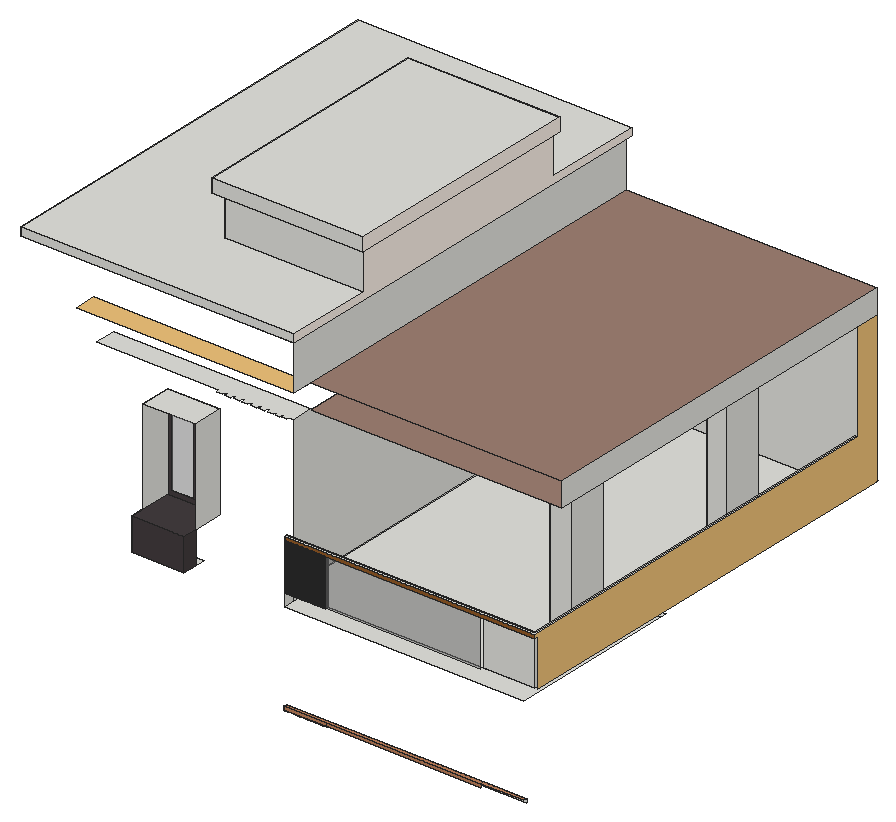
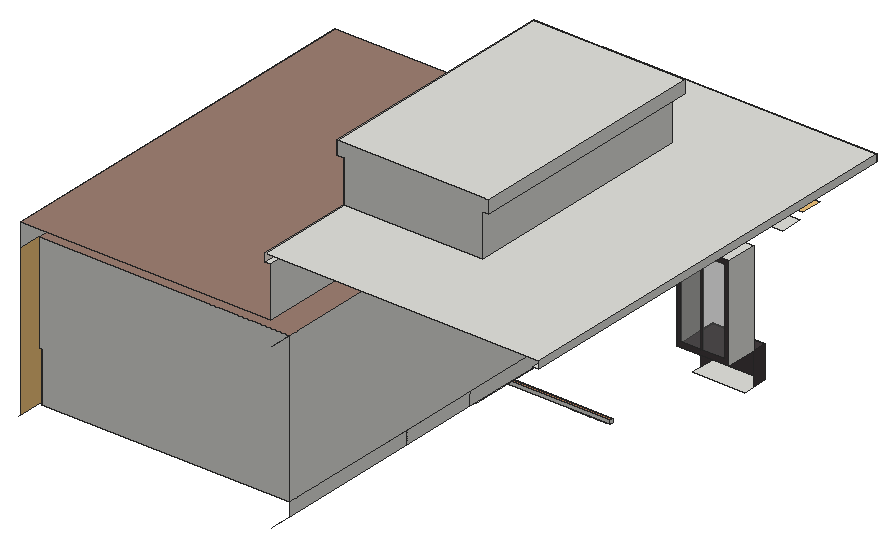
# SketchUp Ruby script. Lengths in inches.
U = 1.inch
M = Sketchup.active_model
def pt(a) = Geom::Point3d.new(a.map { |v| v * U })
def face(e, loops, mat)
  f = e.add_face(loops[0].map { |a| pt(a) })
  loops[1..].each { |l| e.add_face(l.map { |a| pt(a) }).erase! }
  f.material = f.back_material = mat if mat
  f
end
# faces: each face lists its corners as indices into pts; further lists are holes
def faces(e, pts, list, mat = nil) = list.each { |f| face(e, (f[0].is_a?(Array) ? f : [f]).map { |l| l.map { |i| pts[i] } }, mat) }
# xy, xz, yz: faces in a plane at the given z, y or x. An outline is a flat list of corners, or four numbers for a rectangle; further outlines are holes
def ring(l) = l.size == 4 ? [[l[0], l[1]], [l[2], l[1]], [l[2], l[3]], [l[0], l[3]]] : l.each_slice(2).to_a
def flat(e, list, mat, &to3) = list.each { |f| face(e, (f[0].is_a?(Array) ? f : [f]).map { |l| ring(l).map { |u, v| to3.(u, v) } }, mat) }
def xy(e, z, list, mat = nil) = flat(e, list, mat) { |x, y| [x, y, z] }
def xz(e, y, list, mat = nil) = flat(e, list, mat) { |x, z| [x, y, z] }
def yz(e, x, list, mat = nil) = flat(e, list, mat) { |y, z| [x, y, z] }
def lines(e, pts, list) = list.each { |a, b| e.add_line(pt(pts[a]), pt(pts[b])) }
# prism: a flat outline (further loops are holes) pulled along v
def prism(e, loops, v, mat = nil)
  f = face(e, loops, mat); d = Geom::Vector3d.new(v.map { |x| x * U })
  f.pushpull(f.normal.samedirection?(d) ? d.length : -d.length)
end
def box(e, o, s, mat = nil) = prism(e, [[o, [o[0] + s[0], o[1], o[2]], [o[0] + s[0], o[1] + s[1], o[2]], [o[0], o[1] + s[1], o[2]]]], [0, 0, s[2]], mat)
def at(x, y, z, deg = 0) = Geom::Transformation.translation(pt([x, y, z])) * Geom::Transformation.rotation(ORIGIN, Z_AXIS, deg.degrees)
def axes(o, x, y, z) = Geom::Transformation.new([*x, 0, *y, 0, *z, 0, *pt(o).to_a, 1])
def part(name) = M.definitions.add(name)
# library, detail: a bought-in or finely detailed component or shape, given as its bounding box
def library(name, o, s) = part(name).tap { |d| box(d.entities, o, s) }
def detail(e, o, s) = box(e.add_group.entities, o, s)
def put(e, d, t, mat = nil) = e.add_instance(d, t).tap { |i| i.material = mat if mat }
def group(e, t, mat = nil) = e.add_group.tap { |g| g.transformation = t; g.material = mat if mat }.entities
root = M.entities
M.materials.add("Niraj_Skin").color = [158, 128, 115]
M.materials.add("[0009_Linen]").color = [250, 240, 230]
M.materials.add("[Asphalt New]").color = [67, 60, 62]
M.materials.add("[Translucent Glass Gray]").color = [128, 128, 128]
M.materials["[Translucent Glass Gray]"].alpha = 0.5
M.materials.add("[Wood Floor Parquet]").color = [145, 89, 39]
M.materials.add("[Wood OSB]").color = [240, 195, 122]
M.materials.add("[Wood Veneer 02]").color = [190, 128, 91]
xy(root,232.0625,[[228.72,126.77,231.29,127.27],[231.29,126.77,231.72,129.76],[231.72,126.77,233.04,127.39],[233.04,126.77,233.47,129.76],[233.47,126.77,234.79,127.46],
  [234.79,126.77,235.22,129.76],[235.22,126.77,236.54,127.64],[236.54,126.77,236.97,129.76],[236.97,126.77,238.29,127.46],[238.29,126.77,238.72,129.76],
  [238.72,126.77,240.04,127.64],[240.04,126.77,240.47,129.76],[240.47,126.77,241.79,127.33],[241.79,126.77,242.22,129.76],[242.22,126.77,243.54,127.27],
  [243.54,126.77,243.97,129.76],[243.97,126.77,245.29,127.27],[245.29,126.77,245.72,129.76],[245.72,126.77,247.04,127.27],[247.04,126.77,247.54,129.76],
  [247.54,126.77,248.85,127.27],[248.85,126.77,249.35,129.76],[249.35,126.77,250.67,127.27],[250.67,126.77,251.16,129.76],[251.16,126.77,252.48,127.27],
  [252.48,126.77,252.97,129.76],[252.97,126.77,254.29,127.27],[254.29,126.77,254.79,129.76],[254.79,126.77,256.1,127.27],[256.1,126.77,256.6,129.76],
  [256.6,126.77,257.92,127.27],[257.92,126.77,258.41,129.76],[258.41,126.77,259.73,127.27],[259.73,126.77,260.22,129.76],[260.22,126.77,261.54,127.27],
  [261.54,126.77,262.04,129.76],[262.04,126.77,263.35,127.27],[263.35,126.77,263.85,129.76],[263.85,126.77,265.17,127.27],[228.72,127.27,228.75,129.76],
  [228.75,127.27,231.29,129.76],[242.22,127.27,243.54,129.76],[243.97,127.27,245.29,129.76],[245.72,127.27,247.04,129.76],[247.54,127.27,248.85,129.76],
  [249.35,127.27,250.67,129.76],[251.16,127.27,252.48,129.76],[252.97,127.27,254.29,129.76],[254.79,127.27,256.1,129.76],[256.6,127.27,257.92,129.76],
  [258.41,127.27,259.73,129.76],[260.22,127.27,261.54,129.76],[262.04,127.27,263.35,129.76],[240.47,127.33,241.79,129.76],[231.72,127.39,233.04,129.76],
  [233.47,127.46,234.79,129.76],[236.97,127.46,238.29,129.76],[235.22,127.64,236.54,129.76],[238.72,127.64,240.04,129.76]])
xy(root,235.06,[[228.72,126.77,396.96,129.76],[396.96,126.77,433.38,129.76]],"[Wood Veneer 02]")
xy(root,308.65,[[99.93,124.58,144.79,146.21]])
xy(root,311.125,[[228.75,126.77,433.38,272.95],[227.87,136.77,228.75,176.35],[227.87,176.35,228.75,272.95],[228.75,272.95,433.38,278.53]])
xy(root,322.1875,[[228.75,126.77,229.82,127.39],[229.82,126.77,230.22,129.24],[230.22,126.77,230.99,127.39],[230.99,126.77,231.28,129.24],[231.28,126.77,232.05,127.39],
  [232.05,126.77,232.34,129.24],[232.34,126.77,233.11,127.39],[233.11,126.77,233.4,129.24],[233.4,126.77,234.17,127.39],[234.17,126.77,234.47,129.24],
  [234.47,126.77,235.24,127.39],[235.24,126.77,235.53,129.24],[235.53,126.77,236.3,127.39],[236.3,126.77,236.59,129.24],[236.59,126.77,237.36,127.39],
  [237.36,126.77,237.65,129.24],[237.65,126.77,238.42,127.39],[238.42,126.77,238.72,129.24],[238.72,126.77,239.49,127.39],[239.49,126.77,239.78,129.24],
  [239.78,126.77,240.55,127.39],[240.55,126.77,240.84,129.24],[240.84,126.77,241.61,127.39],[241.61,126.77,241.9,129.24],[241.9,126.77,242.67,127.39],
  [242.67,126.77,242.97,129.24],[242.97,126.77,243.74,127.39],[243.74,126.77,244.03,129.24],[244.03,126.77,244.8,127.39],[244.8,126.77,245.09,129.24],
  [245.09,126.77,245.86,127.39],[245.86,126.77,246.15,129.24],[246.15,126.77,246.92,127.39],[246.92,126.77,247.22,129.24],[247.22,126.77,247.99,127.39],
  [247.99,126.77,248.28,129.24],[248.28,126.77,249.05,127.39],[249.05,126.77,249.34,129.24],[249.34,126.77,250.11,127.39],[250.11,126.77,250.4,129.24],
  [250.4,126.77,251.17,127.39],[251.17,126.77,251.47,129.24],[251.47,126.77,252.24,127.39],[252.24,126.77,252.72,129.24],[252.72,126.77,253.49,127.39],
  [253.49,126.77,253.84,129.24],[253.84,126.77,254.61,127.39],[254.61,126.77,255.15,129.24],[255.15,126.77,255.92,127.14],[255.92,126.77,256.4,129.24],
  [256.4,126.77,257.17,127.14],[257.17,126.77,257.78,129.24],[257.78,126.77,258.55,127.14],[258.55,126.77,259.15,129.24],[259.15,126.77,259.92,127.14],
  [259.92,126.77,260.53,129.24],[260.53,126.77,261.3,127.14],[261.3,126.77,261.9,129.24],[261.9,126.77,262.67,127.14],[262.67,126.77,263.28,129.24],
  [255.15,127.14,255.92,129.24],[256.4,127.14,257.17,129.24],[257.78,127.14,258.55,129.24],[259.15,127.14,259.92,129.24],[260.53,127.14,261.3,129.24],
  [261.9,127.14,262.67,129.24],[230.22,127.39,230.99,129.24],[231.28,127.39,232.05,129.24],[232.34,127.39,233.11,129.24],[233.4,127.39,234.17,129.24],
  [234.47,127.39,235.24,129.24],[235.53,127.39,236.3,129.24],[236.59,127.39,237.36,129.24],[237.65,127.39,238.42,129.24],[238.72,127.39,239.49,129.24],
  [239.78,127.39,240.55,129.24],[240.84,127.39,241.61,129.24],[241.9,127.39,242.67,129.24],[242.97,127.39,243.74,129.24],[244.03,127.39,244.8,129.24],
  [245.09,127.39,245.86,129.24],[246.15,127.39,246.92,129.24],[247.22,127.39,247.99,129.24],[248.28,127.39,249.05,129.24],[249.34,127.39,250.11,129.24],
  [250.4,127.39,251.17,129.24],[251.47,127.39,252.24,129.24],[252.72,127.39,253.49,129.24],[253.84,127.39,254.61,129.24],[[228.75,129.24,440.6,471.23],[402.85,193.05,421.1,226.3],[404.6,358.3,421.1,391.55]]])
xy(root,336.38,[[99.93,124.58,144.79,163.21]],"[Asphalt New]")
xy(root,361.9375,[[228.75,126.77,229.82,127.39],[229.82,126.77,230.22,129.24],[230.22,126.77,230.99,127.39],[230.99,126.77,231.28,129.24],[231.28,126.77,232.05,127.39],
  [232.05,126.77,232.34,129.24],[232.34,126.77,233.11,127.39],[233.11,126.77,233.4,129.24],[233.4,126.77,234.17,127.39],[234.17,126.77,234.47,129.24],
  [234.47,126.77,235.24,127.39],[235.24,126.77,235.53,129.24],[235.53,126.77,236.3,127.39],[236.3,126.77,236.59,129.24],[236.59,126.77,237.36,127.39],
  [237.36,126.77,237.65,129.24],[237.65,126.77,238.42,127.39],[238.42,126.77,238.72,129.24],[238.72,126.77,239.49,127.39],[239.49,126.77,239.78,129.24],
  [239.78,126.77,240.55,127.39],[240.55,126.77,240.84,129.24],[240.84,126.77,241.61,127.39],[241.61,126.77,241.9,129.24],[241.9,126.77,242.67,127.39],
  [242.67,126.77,242.97,129.24],[242.97,126.77,243.74,127.39],[243.74,126.77,244.03,129.24],[244.03,126.77,244.8,127.39],[244.8,126.77,245.09,129.24],
  [245.09,126.77,245.86,127.39],[245.86,126.77,246.15,129.24],[246.15,126.77,246.92,127.39],[246.92,126.77,247.22,129.24],[247.22,126.77,247.99,127.39],
  [247.99,126.77,248.28,129.24],[248.28,126.77,249.05,127.39],[249.05,126.77,249.34,129.24],[249.34,126.77,250.11,127.39],[250.11,126.77,250.4,129.24],
  [250.4,126.77,251.17,127.39],[251.17,126.77,251.47,129.24],[251.47,126.77,252.24,127.39],[252.24,126.77,252.72,129.24],[252.72,126.77,253.49,127.39],
  [253.49,126.77,253.84,129.24],[253.84,126.77,254.61,127.39],[254.61,126.77,255.15,129.24],[255.15,126.77,255.92,127.14],[255.92,126.77,256.4,129.24],
  [256.4,126.77,257.17,127.14],[257.17,126.77,257.78,129.24],[257.78,126.77,258.55,127.14],[258.55,126.77,259.15,129.24],[259.15,126.77,259.92,127.14],
  [259.92,126.77,260.53,129.24],[260.53,126.77,261.3,127.14],[261.3,126.77,261.9,129.24],[261.9,126.77,262.67,127.14],[262.67,126.77,263.28,129.24],
  [255.15,127.14,255.92,129.24],[256.4,127.14,257.17,129.24],[257.78,127.14,258.55,129.24],[259.15,127.14,259.92,129.24],[260.53,127.14,261.3,129.24],
  [261.9,127.14,262.67,129.24],[228.75,127.39,229.82,129.24],[230.22,127.39,230.99,129.24],[231.28,127.39,232.05,129.24],[232.34,127.39,233.11,129.24],
  [233.4,127.39,234.17,129.24],[234.47,127.39,235.24,129.24],[235.53,127.39,236.3,129.24],[236.59,127.39,237.36,129.24],[237.65,127.39,238.42,129.24],
  [238.72,127.39,239.49,129.24],[239.78,127.39,240.55,129.24],[240.84,127.39,241.61,129.24],[241.9,127.39,242.67,129.24],[242.97,127.39,243.74,129.24],
  [244.03,127.39,244.8,129.24],[245.09,127.39,245.86,129.24],[246.15,127.39,246.92,129.24],[247.22,127.39,247.99,129.24],[248.28,127.39,249.05,129.24],
  [249.34,127.39,250.11,129.24],[250.4,127.39,251.17,129.24],[251.47,127.39,252.24,129.24],[252.72,127.39,253.49,129.24],[253.84,127.39,254.61,129.24]])
xy(root,364.9375,[[228.75,126.77,443,126.77,443,471.23,440.6,471.23,440.6,129.24,228.75,129.24]])
xy(root,416.99,[[99.93,136.77,144.79,163.21]])
xy(root,449.78,[[228.75,154.83,443,471.23]],"Niraj_Skin")
xy(root,450.1,[[164.91,134.14,170.31,134.14,170.31,136.77,172.16,136.77,172.16,134.14,177.56,134.14,177.56,136.77,179.41,136.77,179.41,134.14,184.81,134.14,184.81,136.77,186.66,136.77,186.66,134.14,192.06,134.14,192.06,136.77,193.91,136.77,193.91,134.14,199.31,134.14,199.31,136.77,201.16,136.77,201.16,134.14,206.56,134.14,206.56,136.77,208.41,136.77,208.41,134.14,213.81,134.14,213.81,136.77,215.35,136.77,215.35,134.14,219.35,134.14,219.35,136.77,220.74,136.77,220.74,134.14,224.75,134.14,224.75,136.77,228.75,136.77,228.75,154.83,60.84,154.83,60.84,136.77,164.91,136.77]])
xy(root,451.75,[[402.85,193.05,421.1,226.3]])
xy(root,452.25,[[404.6,358.3,421.1,391.55]])
xy(root,470.41,[[228.75,154.83,443,490.875]],"Niraj_Skin")
xy(root,470.41,[[43.27,136.77,228.75,154.83]],"[Wood OSB]")
xy(root,513.13,[[0,130.89,5.25,490.875],[5.25,130.89,233.81,136.77],[228.75,136.77,233.81,490.875]])
xy(root,519.625,[[0,130.89,233.81,130.89,233.81,204.9,115.81,204.9,115.81,406.59,233.81,406.59,233.81,490.875,0,490.875]])
xy(root,555.58,[[110.5,197.09,115.81,406.59],[115.81,197.09,233.81,204.9]])
xy(root,555.58,[[233.81,197.09,239.87,406.59]],"[0009_Linen]")
xy(root,566.8125,[[110.5,197.09,239.87,406.59]])
xz(root,124.58,[[99.93,308.65,144.79,336.38]],"[Asphalt New]")
xz(root,126.77,[[264.05,322.1875,396.96,361.9375]],"[Translucent Glass Gray]")
xz(root,126.77,[[229.82,322.1875,230.22,361.9375],[230.99,322.1875,231.28,361.9375],[232.05,322.1875,232.34,361.9375],[233.11,322.1875,233.4,361.9375],[234.17,322.1875,234.47,361.9375],
  [235.24,322.1875,235.53,361.9375],[236.3,322.1875,236.59,361.9375],[237.36,322.1875,237.65,361.9375],[238.42,322.1875,238.72,361.9375],[239.49,322.1875,239.78,361.9375],
  [240.55,322.1875,240.84,361.9375],[241.61,322.1875,241.9,361.9375],[242.67,322.1875,242.97,361.9375],[243.74,322.1875,244.03,361.9375],[244.8,322.1875,245.09,361.9375],
  [245.86,322.1875,246.15,361.9375],[246.92,322.1875,247.22,361.9375],[247.99,322.1875,248.28,361.9375],[249.05,322.1875,249.34,361.9375],[250.11,322.1875,250.4,361.9375],
  [251.17,322.1875,251.47,361.9375],[252.24,322.1875,252.72,361.9375],[253.49,322.1875,253.84,361.9375],[254.61,322.1875,255.15,361.9375],[255.92,322.1875,256.4,361.9375],
  [257.17,322.1875,257.78,361.9375],[258.55,322.1875,259.15,361.9375],[259.92,322.1875,260.53,361.9375],[261.3,322.1875,261.9,361.9375],[262.67,322.1875,263.28,361.9375],
  [263.28,322.1875,264.05,361.9375],[228.75,361.9375,443,364.9375]],"[Wood Floor Parquet]")
xz(root,126.77,[[228.72,232.0625,263.85,235.06],[263.85,232.0625,396.96,235.06]],"[Wood Veneer 02]")
xz(root,127.14,[[255.15,322.1875,255.92,361.9375],[256.4,322.1875,257.17,361.9375],[257.78,322.1875,258.55,361.9375],[259.15,322.1875,259.92,361.9375],[260.53,322.1875,261.3,361.9375],
  [261.9,322.1875,262.67,361.9375]],"[Wood Floor Parquet]")
xz(root,127.39,[[228.75,322.1875,229.82,361.9375]])
xz(root,127.39,[[230.22,322.1875,230.99,361.9375],[231.28,322.1875,232.05,361.9375],[232.34,322.1875,233.11,361.9375],[233.4,322.1875,234.17,361.9375],[234.47,322.1875,235.24,361.9375],
  [235.53,322.1875,236.3,361.9375],[236.59,322.1875,237.36,361.9375],[237.65,322.1875,238.42,361.9375],[238.72,322.1875,239.49,361.9375],[239.78,322.1875,240.55,361.9375],
  [240.84,322.1875,241.61,361.9375],[241.9,322.1875,242.67,361.9375],[242.97,322.1875,243.74,361.9375],[244.03,322.1875,244.8,361.9375],[245.09,322.1875,245.86,361.9375],
  [246.15,322.1875,246.92,361.9375],[247.22,322.1875,247.99,361.9375],[248.28,322.1875,249.05,361.9375],[249.34,322.1875,250.11,361.9375],[250.4,322.1875,251.17,361.9375],
  [251.47,322.1875,252.24,361.9375],[252.72,322.1875,253.49,361.9375],[253.84,322.1875,254.61,361.9375]],"[Wood Floor Parquet]")
xz(root,129.24,[[228.75,322.1875,229.82,361.9375],[230.22,322.1875,230.99,361.9375],[231.28,322.1875,232.05,361.9375],[232.34,322.1875,233.11,361.9375],[233.4,322.1875,234.17,361.9375],
  [234.47,322.1875,235.24,361.9375],[235.53,322.1875,236.3,361.9375],[236.59,322.1875,237.36,361.9375],[237.65,322.1875,238.42,361.9375],[238.72,322.1875,239.49,361.9375],
  [239.78,322.1875,240.55,361.9375],[240.84,322.1875,241.61,361.9375],[241.9,322.1875,242.67,361.9375],[242.97,322.1875,243.74,361.9375],[244.03,322.1875,244.8,361.9375],
  [245.09,322.1875,245.86,361.9375],[246.15,322.1875,246.92,361.9375],[247.22,322.1875,247.99,361.9375],[248.28,322.1875,249.05,361.9375],[249.34,322.1875,250.11,361.9375],
  [250.4,322.1875,251.17,361.9375],[251.47,322.1875,252.24,361.9375],[252.72,322.1875,253.49,361.9375],[253.84,322.1875,254.61,361.9375],[255.15,322.1875,255.92,361.9375],
  [256.4,322.1875,257.17,361.9375],[257.78,322.1875,258.55,361.9375],[259.15,322.1875,259.92,361.9375],[260.53,322.1875,261.3,361.9375],[261.9,322.1875,262.67,361.9375],
  [263.28,322.1875,264.05,361.9375],[396.96,322.1875,440.6,361.9375],[228.75,361.9375,440.6,364.9375]])
xz(root,129.76,[[228.72,232.0625,433.38,235.06]])
xz(root,130.89,[[0,513.13,233.81,519.625]])
xz(root,163.21,[[[99.93,336.38,144.79,416.99],[103.82,340.27,140.91,413.1]],[122.36,340.27,124.29,413.1]],"[Asphalt New]")
xz(root,163.21,[[103.82,340.27,122.36,413.1],[124.29,340.27,140.91,413.1]],"[Translucent Glass Gray]")
xz(root,193.05,[[402.85,322.1875,421.1,451.75]])
xz(root,197.09,[[110.5,555.58,239.87,566.8125]])
xz(root,204.9,[[115.81,519.625,233.81,555.58]])
xz(root,226.3,[[402.85,322.1875,421.1,451.75]])
xz(root,358.3,[[404.6,322.1875,421.1,452.25]])
xz(root,391.55,[[404.6,322.1875,421.1,452.25]])
xz(root,406.59,[[115.81,519.625,115.81,555.58,110.5,555.58,110.5,566.8125,239.87,566.8125,239.87,555.58,233.81,555.58,233.81,519.625]])
xz(root,471.23,[[228.75,322.1875,440.6,322.1875,440.6,364.9375,443,364.9375,443,449.78,228.75,449.78]])
yz(root,0,[[130.89,513.13,490.875,519.625]])
yz(root,99.93,[[136.77,336.38,163.21,416.99]])
yz(root,99.93,[[124.58,308.65,136.77,336.38]],"[Asphalt New]")
yz(root,110.5,[[197.09,555.58,406.59,566.8125]])
yz(root,115.81,[[204.9,519.625,406.59,555.58]])
yz(root,144.79,[[136.77,336.38,163.21,416.99]])
yz(root,144.79,[[124.58,308.65,136.77,336.38]],"[Asphalt New]")
yz(root,228.72,[[126.77,232.0625,129.76,235.06]])
yz(root,228.75,[[126.77,311.125,126.77,322.1875,127.39,322.1875,127.39,361.9375,129.24,361.9375,129.24,322.1875,136.77,322.1875,136.77,311.125],[136.77,311.125,176.35,322.1875],[176.35,311.125,278.53,322.1875],[278.53,311.125,346.4375,322.1875],[346.4375,311.125,471.23,322.1875],
  [136.77,322.1875,471.23,322.1875,471.23,449.78,154.83,449.78,154.83,450.1,136.77,450.1],[126.77,361.9375,129.24,364.9375],[136.77,470.41,490.875,513.13]])
yz(root,229.82,[[127.39,322.1875,129.24,361.9375]])
yz(root,229.82,[[126.77,322.1875,127.39,361.9375]],"[Wood Floor Parquet]")
yz(root,230.22,[[127.39,322.1875,129.24,361.9375]])
yz(root,230.22,[[126.77,322.1875,127.39,361.9375]],"[Wood Floor Parquet]")
yz(root,230.99,[[127.39,322.1875,129.24,361.9375]])
yz(root,230.99,[[126.77,322.1875,127.39,361.9375]],"[Wood Floor Parquet]")
yz(root,231.28,[[127.39,322.1875,129.24,361.9375]])
yz(root,231.28,[[126.77,322.1875,127.39,361.9375]],"[Wood Floor Parquet]")
yz(root,232.05,[[127.39,322.1875,129.24,361.9375]])
yz(root,232.05,[[126.77,322.1875,127.39,361.9375]],"[Wood Floor Parquet]")
yz(root,232.34,[[127.39,322.1875,129.24,361.9375]])
yz(root,232.34,[[126.77,322.1875,127.39,361.9375]],"[Wood Floor Parquet]")
yz(root,233.11,[[127.39,322.1875,129.24,361.9375]])
yz(root,233.11,[[126.77,322.1875,127.39,361.9375]],"[Wood Floor Parquet]")
yz(root,233.4,[[127.39,322.1875,129.24,361.9375]])
yz(root,233.4,[[126.77,322.1875,127.39,361.9375]],"[Wood Floor Parquet]")
yz(root,233.81,[[130.89,513.13,490.875,513.13,490.875,519.625,406.59,519.625,406.59,555.58,204.9,555.58,204.9,519.625,130.89,519.625]],"[0009_Linen]")
yz(root,234.17,[[127.39,322.1875,129.24,361.9375]])
yz(root,234.17,[[126.77,322.1875,127.39,361.9375]],"[Wood Floor Parquet]")
yz(root,234.47,[[127.39,322.1875,129.24,361.9375]])
yz(root,234.47,[[126.77,322.1875,127.39,361.9375]],"[Wood Floor Parquet]")
yz(root,235.24,[[127.39,322.1875,129.24,361.9375]])
yz(root,235.24,[[126.77,322.1875,127.39,361.9375]],"[Wood Floor Parquet]")
yz(root,235.53,[[127.39,322.1875,129.24,361.9375]])
yz(root,235.53,[[126.77,322.1875,127.39,361.9375]],"[Wood Floor Parquet]")
yz(root,236.3,[[127.39,322.1875,129.24,361.9375]])
yz(root,236.3,[[126.77,322.1875,127.39,361.9375]],"[Wood Floor Parquet]")
yz(root,236.59,[[127.39,322.1875,129.24,361.9375]])
yz(root,236.59,[[126.77,322.1875,127.39,361.9375]],"[Wood Floor Parquet]")
yz(root,237.36,[[127.39,322.1875,129.24,361.9375]])
yz(root,237.36,[[126.77,322.1875,127.39,361.9375]],"[Wood Floor Parquet]")
yz(root,237.65,[[127.39,322.1875,129.24,361.9375]])
yz(root,237.65,[[126.77,322.1875,127.39,361.9375]],"[Wood Floor Parquet]")
yz(root,238.42,[[127.39,322.1875,129.24,361.9375]])
yz(root,238.42,[[126.77,322.1875,127.39,361.9375]],"[Wood Floor Parquet]")
yz(root,238.72,[[127.39,322.1875,129.24,361.9375]])
yz(root,238.72,[[126.77,322.1875,127.39,361.9375]],"[Wood Floor Parquet]")
yz(root,239.49,[[127.39,322.1875,129.24,361.9375]])
yz(root,239.49,[[126.77,322.1875,127.39,361.9375]],"[Wood Floor Parquet]")
yz(root,239.78,[[127.39,322.1875,129.24,361.9375]])
yz(root,239.78,[[126.77,322.1875,127.39,361.9375]],"[Wood Floor Parquet]")
yz(root,239.87,[[197.09,555.58,406.59,566.8125]],"[0009_Linen]")
yz(root,240.55,[[127.39,322.1875,129.24,361.9375]])
yz(root,240.55,[[126.77,322.1875,127.39,361.9375]],"[Wood Floor Parquet]")
yz(root,240.84,[[127.39,322.1875,129.24,361.9375]])
yz(root,240.84,[[126.77,322.1875,127.39,361.9375]],"[Wood Floor Parquet]")
yz(root,241.61,[[127.39,322.1875,129.24,361.9375]])
yz(root,241.61,[[126.77,322.1875,127.39,361.9375]],"[Wood Floor Parquet]")
yz(root,241.9,[[127.39,322.1875,129.24,361.9375]])
yz(root,241.9,[[126.77,322.1875,127.39,361.9375]],"[Wood Floor Parquet]")
yz(root,242.67,[[127.39,322.1875,129.24,361.9375]])
yz(root,242.67,[[126.77,322.1875,127.39,361.9375]],"[Wood Floor Parquet]")
yz(root,242.97,[[127.39,322.1875,129.24,361.9375]])
yz(root,242.97,[[126.77,322.1875,127.39,361.9375]],"[Wood Floor Parquet]")
yz(root,243.74,[[127.39,322.1875,129.24,361.9375]])
yz(root,243.74,[[126.77,322.1875,127.39,361.9375]],"[Wood Floor Parquet]")
yz(root,244.03,[[127.39,322.1875,129.24,361.9375]])
yz(root,244.03,[[126.77,322.1875,127.39,361.9375]],"[Wood Floor Parquet]")
yz(root,244.8,[[127.39,322.1875,129.24,361.9375]])
yz(root,244.8,[[126.77,322.1875,127.39,361.9375]],"[Wood Floor Parquet]")
yz(root,245.09,[[127.39,322.1875,129.24,361.9375]])
yz(root,245.09,[[126.77,322.1875,127.39,361.9375]],"[Wood Floor Parquet]")
yz(root,245.86,[[127.39,322.1875,129.24,361.9375]])
yz(root,245.86,[[126.77,322.1875,127.39,361.9375]],"[Wood Floor Parquet]")
yz(root,246.15,[[127.39,322.1875,129.24,361.9375]])
yz(root,246.15,[[126.77,322.1875,127.39,361.9375]],"[Wood Floor Parquet]")
yz(root,246.92,[[127.39,322.1875,129.24,361.9375]])
yz(root,246.92,[[126.77,322.1875,127.39,361.9375]],"[Wood Floor Parquet]")
yz(root,247.22,[[127.39,322.1875,129.24,361.9375]])
yz(root,247.22,[[126.77,322.1875,127.39,361.9375]],"[Wood Floor Parquet]")
yz(root,247.99,[[127.39,322.1875,129.24,361.9375]])
yz(root,247.99,[[126.77,322.1875,127.39,361.9375]],"[Wood Floor Parquet]")
yz(root,248.28,[[127.39,322.1875,129.24,361.9375]])
yz(root,248.28,[[126.77,322.1875,127.39,361.9375]],"[Wood Floor Parquet]")
yz(root,249.05,[[127.39,322.1875,129.24,361.9375]])
yz(root,249.05,[[126.77,322.1875,127.39,361.9375]],"[Wood Floor Parquet]")
yz(root,249.34,[[127.39,322.1875,129.24,361.9375]])
yz(root,249.34,[[126.77,322.1875,127.39,361.9375]],"[Wood Floor Parquet]")
yz(root,250.11,[[127.39,322.1875,129.24,361.9375]])
yz(root,250.11,[[126.77,322.1875,127.39,361.9375]],"[Wood Floor Parquet]")
yz(root,250.4,[[127.39,322.1875,129.24,361.9375]])
yz(root,250.4,[[126.77,322.1875,127.39,361.9375]],"[Wood Floor Parquet]")
yz(root,251.17,[[127.39,322.1875,129.24,361.9375]])
yz(root,251.17,[[126.77,322.1875,127.39,361.9375]],"[Wood Floor Parquet]")
yz(root,251.47,[[127.39,322.1875,129.24,361.9375]])
yz(root,251.47,[[126.77,322.1875,127.39,361.9375]],"[Wood Floor Parquet]")
yz(root,252.24,[[127.39,322.1875,129.24,361.9375]])
yz(root,252.24,[[126.77,322.1875,127.39,361.9375]],"[Wood Floor Parquet]")
yz(root,252.72,[[127.39,322.1875,129.24,361.9375]])
yz(root,252.72,[[126.77,322.1875,127.39,361.9375]],"[Wood Floor Parquet]")
yz(root,253.49,[[127.39,322.1875,129.24,361.9375]])
yz(root,253.49,[[126.77,322.1875,127.39,361.9375]],"[Wood Floor Parquet]")
yz(root,253.84,[[127.39,322.1875,129.24,361.9375]])
yz(root,253.84,[[126.77,322.1875,127.39,361.9375]],"[Wood Floor Parquet]")
yz(root,254.61,[[127.39,322.1875,129.24,361.9375]])
yz(root,254.61,[[126.77,322.1875,127.39,361.9375]],"[Wood Floor Parquet]")
yz(root,255.15,[[127.14,322.1875,129.24,361.9375]])
yz(root,255.15,[[126.77,322.1875,127.14,361.9375]],"[Wood Floor Parquet]")
yz(root,255.92,[[127.14,322.1875,129.24,361.9375]])
yz(root,255.92,[[126.77,322.1875,127.14,361.9375]],"[Wood Floor Parquet]")
yz(root,256.4,[[127.14,322.1875,129.24,361.9375]])
yz(root,256.4,[[126.77,322.1875,127.14,361.9375]],"[Wood Floor Parquet]")
yz(root,257.17,[[127.14,322.1875,129.24,361.9375]])
yz(root,257.17,[[126.77,322.1875,127.14,361.9375]],"[Wood Floor Parquet]")
yz(root,257.78,[[127.14,322.1875,129.24,361.9375]])
yz(root,257.78,[[126.77,322.1875,127.14,361.9375]],"[Wood Floor Parquet]")
yz(root,258.55,[[127.14,322.1875,129.24,361.9375]])
yz(root,258.55,[[126.77,322.1875,127.14,361.9375]],"[Wood Floor Parquet]")
yz(root,259.15,[[127.14,322.1875,129.24,361.9375]])
yz(root,259.15,[[126.77,322.1875,127.14,361.9375]],"[Wood Floor Parquet]")
yz(root,259.92,[[127.14,322.1875,129.24,361.9375]])
yz(root,259.92,[[126.77,322.1875,127.14,361.9375]],"[Wood Floor Parquet]")
yz(root,260.53,[[127.14,322.1875,129.24,361.9375]])
yz(root,260.53,[[126.77,322.1875,127.14,361.9375]],"[Wood Floor Parquet]")
yz(root,261.3,[[127.14,322.1875,129.24,361.9375]])
yz(root,261.3,[[126.77,322.1875,127.14,361.9375]],"[Wood Floor Parquet]")
yz(root,261.9,[[127.14,322.1875,129.24,361.9375]])
yz(root,261.9,[[126.77,322.1875,127.14,361.9375]],"[Wood Floor Parquet]")
yz(root,262.67,[[127.14,322.1875,129.24,361.9375]])
yz(root,262.67,[[126.77,322.1875,127.14,361.9375]],"[Wood Floor Parquet]")
yz(root,263.28,[[126.77,322.1875,129.24,361.9375]])
yz(root,402.85,[[193.05,322.1875,226.3,451.75]])
yz(root,404.6,[[358.3,322.1875,391.55,452.25]])
yz(root,421.1,[[193.05,322.1875,226.3,451.75],[358.3,322.1875,391.55,452.25]])
yz(root,440.6,[[129.24,322.1875,471.23,364.9375]])
yz(root,443,[[154.83,449.78,490.875,470.41]])
yz(root,443,[[129.24,322.1875,490.875,322.1875,490.875,449.78,471.23,449.78,471.23,364.9375,126.77,364.9375,126.77,361.9375,129.24,361.9375]],"[Wood OSB]")
p = [[230.39,126.77,232.0625],[229.97,126.77,232.0625],[229.97,126.28,232.05],[230.39,126.28,232.05],[228.75,490.875,311.125],[228.75,471.23,311.125],
  [228.75,471.23,449.78],[228.75,490.875,449.78],[443,490.875,322.1875],[443,492.62,322.1875]]
faces(root,p,[[0,1,2,3]],"[Wood Floor Parquet]")
lines(root,p,[[4,5],[6,7],[8,9]])
